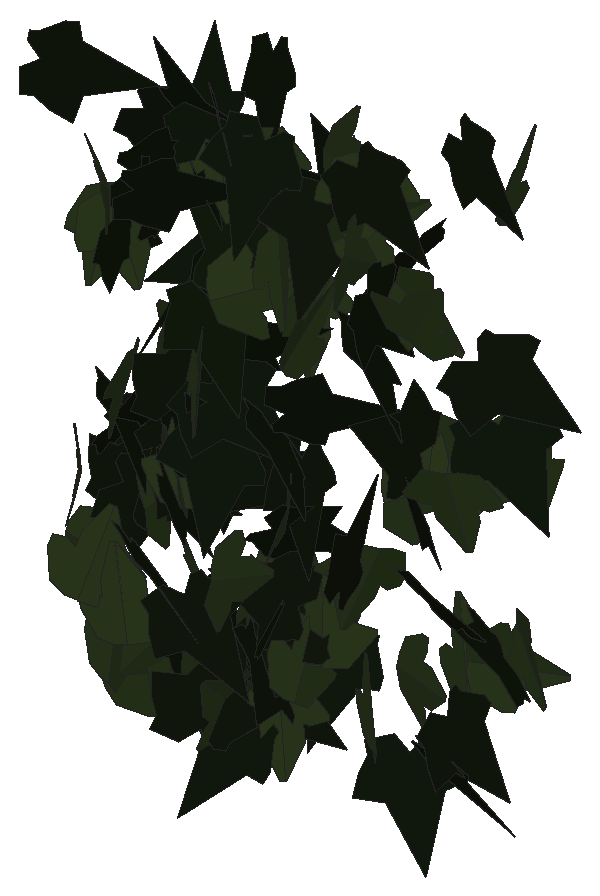
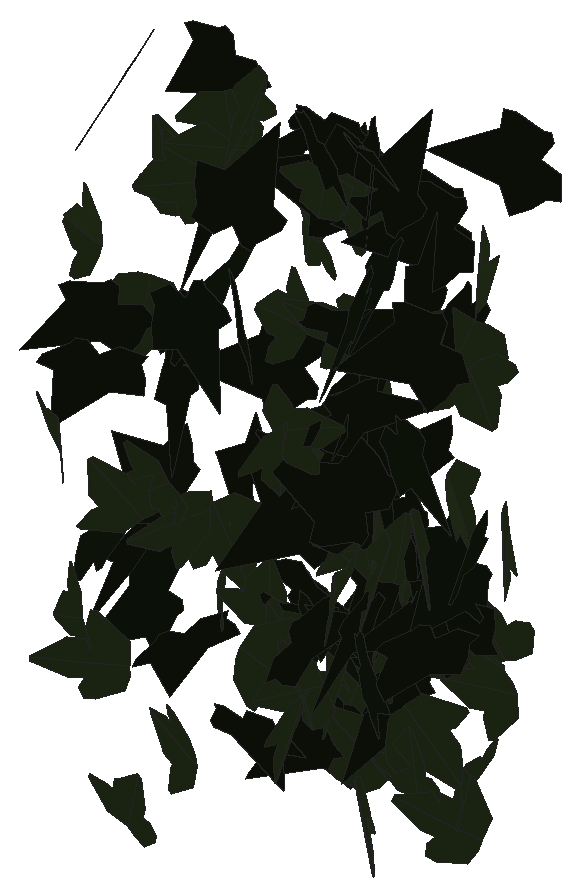
# SketchUp Ruby script. Lengths in inches.
U = 1.inch
M = Sketchup.active_model
def pt(a) = Geom::Point3d.new(a.map { |v| v * U })
def face(e, loops, mat)
  f = e.add_face(loops[0].map { |a| pt(a) })
  loops[1..].each { |l| e.add_face(l.map { |a| pt(a) }).erase! }
  f.material = f.back_material = mat if mat
  f
end
# faces: each face lists its corners as indices into pts; further lists are holes
def faces(e, pts, list, mat = nil) = list.each { |f| face(e, (f[0].is_a?(Array) ? f : [f]).map { |l| l.map { |i| pts[i] } }, mat) }
# xy, xz, yz: faces in a plane at the given z, y or x. An outline is a flat list of corners, or four numbers for a rectangle; further outlines are holes
def ring(l) = l.size == 4 ? [[l[0], l[1]], [l[2], l[1]], [l[2], l[3]], [l[0], l[3]]] : l.each_slice(2).to_a
def flat(e, list, mat, &to3) = list.each { |f| face(e, (f[0].is_a?(Array) ? f : [f]).map { |l| ring(l).map { |u, v| to3.(u, v) } }, mat) }
def xy(e, z, list, mat = nil) = flat(e, list, mat) { |x, y| [x, y, z] }
def xz(e, y, list, mat = nil) = flat(e, list, mat) { |x, z| [x, y, z] }
def yz(e, x, list, mat = nil) = flat(e, list, mat) { |y, z| [x, y, z] }
def lines(e, pts, list) = list.each { |a, b| e.add_line(pt(pts[a]), pt(pts[b])) }
# prism: a flat outline (further loops are holes) pulled along v
def prism(e, loops, v, mat = nil)
  f = face(e, loops, mat); d = Geom::Vector3d.new(v.map { |x| x * U })
  f.pushpull(f.normal.samedirection?(d) ? d.length : -d.length)
end
def box(e, o, s, mat = nil) = prism(e, [[o, [o[0] + s[0], o[1], o[2]], [o[0] + s[0], o[1] + s[1], o[2]], [o[0], o[1] + s[1], o[2]]]], [0, 0, s[2]], mat)
def at(x, y, z, deg = 0) = Geom::Transformation.translation(pt([x, y, z])) * Geom::Transformation.rotation(ORIGIN, Z_AXIS, deg.degrees)
def axes(o, x, y, z) = Geom::Transformation.new([*x, 0, *y, 0, *z, 0, *pt(o).to_a, 1])
def part(name) = M.definitions.add(name)
# library, detail: a bought-in or finely detailed component or shape, given as its bounding box
def library(name, o, s) = part(name).tap { |d| box(d.entities, o, s) }
def detail(e, o, s) = box(e.add_group.entities, o, s)
def put(e, d, t, mat = nil) = e.add_instance(d, t).tap { |i| i.material = mat if mat }
def group(e, t, mat = nil) = e.add_group.tap { |g| g.transformation = t; g.material = mat if mat }.entities
root = M.entities
M.materials.add("efeu1").color = [18, 25, 13]
M.materials.add("efeu2").color = [43, 57, 29]
c1 = part("ivyleaf_9")
p = [[1.54,2.16,1.25],[1.36,2.04,1.19],[-0.21,0.99,0.68],[-0.71,1.11,0.82],[-0.85,0.86,0.67],[-0.8,0.17,0.21],
  [-0.9,-0.01,0.1],[-0.67,-0.16,-0.02],[-0.08,-0.08,-0.05],[-0.03,-0.6,-0.4],[0.65,-0.88,-0.66],[0.83,-0.6,-0.49],
  [1.29,-0.42,-0.43],[1.8125,-0.07,-0.26],[1.21,0.44,0.15]]
faces(c1.entities,p,[[0,1,2,3,4,5,6,7,8,9,10,11,12,13,14]],"efeu1")
c2 = part("ivyleaf_10")
p = [[0,0.5,-0.03],[-0.0625,2.02,-0.43],[-0.19,2.01,-0.46],[-0.54,1.05,-0.29],[-0.52,0.625,-0.18],[-0.83,0.76,-0.28],
  [-1.16,0.64,-0.33],[-1.15,0.33,-0.24],[-0.77,-0.39,0.02],[-0.3,-0.51,0.16],[0.04,-0.48,0.23],[-0.02,2.01,-0.4375],
  [-0.06,2.01,-0.43],[0.04,-0.49,0.23],[0.67,-0.49,0.14],[1.38,0.36,-0.2],[1.375,0.51,-0.24],[0.81,0.65,-0.19],
  [0.62,0.59,-0.15],[0.6,1.09,-0.28],[0.5,1.23,-0.31]]
faces(c2.entities,p,[[0,1,2,3,4,5,6,7,8,9,10],[11,12,0,13,14,15,16,17,18,19,20]],"efeu2")
put(root,c1,axes([37.89,224.72,217.01],[0.06828,-0.29267,-0.3996],[0.02885,0.40505,-0.29173],[0.49447,0.01679,0.0722]))
put(root,c2,axes([38.07,223.66,220.32],[0.25896,0.39819,-0.15615],[-0.07769,-0.13571,-0.47492],[-0.4206,0.27023,-0.00841]))
put(root,c2,axes([38.36,223.23,214.16],[0.00126,0.31534,-0.38802],[-0.07703,0.38351,0.31143],[0.49403,0.05899,0.04955]))
put(root,c2,axes([37.9,223.36,215.67],[-0.1061,-0.00591,-0.48858],[0.46752,-0.14654,-0.09976],[-0.14201,-0.47801,0.03662]))
put(root,c2,axes([38.43,224.34,218.27],[0.23981,-0.31066,-0.30981],[-0.16582,0.26271,-0.39178],[0.4062,0.29065,0.02298]))
put(root,c1,axes([38.34,223.5,217.45],[0.13194,0.388,0.28644],[0.09321,0.27085,-0.40982],[-0.47318,0.16154,-0.00086]))
put(root,c1,axes([37.98,224.53,221.21],[0.05891,0.07528,-0.49078],[0.31473,0.37659,0.09554],[0.38402,-0.32018,-0.00302]))
put(root,c1,axes([38.24,225.7,216.92],[-0.25111,0.04925,-0.42955],[0.39721,-0.16992,-0.25169],[-0.17078,-0.46765,0.04621]))
put(root,c2,axes([38.59,222.34,217.34],[0.11945,-0.23218,-0.42641],[-0.16922,0.39168,-0.26068],[0.45508,0.20659,0.01499]))
put(root,c1,axes([38.09,222.35,222.93],[0.22534,0.05977,-0.44232],[0.26473,0.38104,0.18635],[0.35936,-0.31818,0.14008]))
put(root,c1,axes([38.19,223.74,217.46],[0.16614,-0.37636,0.28417],[0.11736,-0.25881,-0.41139],[0.45675,0.2034,0.00235]))
put(root,c2,axes([38.18,223.69,213.68],[-0.11724,-0.15903,0.45931],[0.41144,0.21909,0.18088],[-0.25879,0.42037,0.07949]))
put(root,c2,axes([38.56,223.4,218.38],[0.19224,-0.45308,0.08813],[0.04208,-0.07787,-0.4921],[0.45965,0.19662,0.00819]))
put(root,c1,axes([38.45,223.53,216.39],[-0.3181,0.09077,0.37494],[0.31904,-0.21129,0.32182],[0.21686,0.44398,0.07651]))
put(root,c2,axes([38.53,222.94,221.02],[-0.266,0.14555,0.39757],[0.31073,-0.25179,0.30008],[0.28756,0.40672,0.0435]))
put(root,c2,axes([38.57,222.53,215.71],[0.40715,0.22638,-0.1816],[0.15911,0.08754,0.46586],[0.24271,-0.43714,-0.00075]))
put(root,c1,axes([38.8,222.83,220.69],[0.06508,-0.02692,-0.49502],[-0.34481,0.35626,-0.0647],[0.35619,0.34979,0.02781]))
put(root,c1,axes([38.87,224.16,219.36],[-0.33398,0.30789,-0.20895],[0.15546,-0.13964,-0.45424],[-0.33807,-0.36838,-0.00246]))
put(root,c2,axes([38.52,223.15,220.61],[0.41422,0.19482,0.20116],[0.17576,0.09875,-0.45755],[-0.21801,0.44977,0.01332]))
put(root,c1,axes([38.5,223.47,216.62],[0.12107,0.03791,-0.48364],[0.13119,0.47734,0.07025],[0.46705,-0.1439,0.10563]))
put(root,c2,axes([38.95,224.82,214.375],[0.18786,-0.30213,-0.35132],[-0.19064,0.29513,-0.35574],[0.42233,0.26761,-0.00431]))
put(root,c2,axes([38.81,223.55,216.45],[0.12865,-0.02468,-0.48253],[0.0261,0.49897,-0.01856],[0.48246,-0.02041,0.12968]))
put(root,c2,axes([39.14,223.51,214.83],[-0.30526,-0.23645,0.31766],[-0.25376,-0.19111,-0.38611],[0.30401,-0.39695,-0.00333]))
put(root,c2,axes([39.12,222.64,215.25],[0.44305,0.21822,0.078],[-0.07088,-0.03261,0.49387],[0.22064,-0.44868,0.00204]))
put(root,c2,axes([39.08,223.61,213.99],[0.49527,-0.04984,0.04714],[-0.04691,0.00468,0.49777],[-0.05006,-0.49749,-0.00004]))
put(root,c2,axes([39.3,224.87,217.23],[-0.06855,0.33915,-0.36094],[-0.1058,0.34595,0.34515],[0.48385,0.1237,0.02434]))
put(root,c1,axes([39.11,223.39,220.84],[0.03874,0.18578,0.46258],[-0.14418,-0.43997,0.18878],[0.47719,-0.14802,0.01948]))
put(root,c1,axes([39.12,224.59,221.51],[0.34556,-0.18671,-0.30941],[-0.27171,0.14801,-0.39277],[0.23826,0.43958,0.00083]))
put(root,c2,axes([39.24,223.51,216.83],[-0.40564,0.28083,0.08119],[0.06484,-0.04899,0.49335],[0.28505,0.41078,0.00332]))
put(root,c1,axes([39.25,224.4,216.82],[0.19395,-0.12326,-0.44406],[-0.29917,0.33279,-0.22304],[0.35054,0.35222,0.05534]))
put(root,c1,axes([39.44,224.75,219.78],[-0.00126,-0.22965,-0.44414],[-0.02405,-0.4436,0.22944],[-0.49942,0.02194,-0.00993]))
put(root,c1,axes([39.28,223.24,217.05],[0.35864,-0.15511,-0.31196],[-0.27416,0.15061,-0.39007],[0.21498,0.45084,0.02298]))
put(root,c2,axes([39.49,223.77,217.21],[-0.14057,0.22616,0.42319],[-0.24515,0.34523,-0.26593],[-0.41248,-0.28225,0.01383]))
put(root,c1,axes([38.96,223.63,217.67],[0.15554,-0.09957,-0.46464],[0.47489,0.04995,0.14826],[0.01689,-0.48743,0.11011]))
put(root,c1,axes([39.49,223.4375,215.13],[-0.00738,0.01927,-0.49957],[-0.28837,0.40797,0.02],[0.4084,0.28842,0.00509]))
put(root,c1,axes([39.24,222.68,221.64],[0.07634,0.2977,-0.39439],[0.01251,0.39778,0.30268],[0.49398,-0.05608,0.05328]))
put(root,c2,axes([39.47,223.47,216.93],[0.41651,0.2713,0.05402],[-0.05339,-0.01696,0.49685],[0.27142,-0.41965,0.01483]))
put(root,c1,axes([39.5,223.77,220.15],[0.15808,-0.0587,-0.47071],[-0.34269,0.32893,-0.15611],[0.32799,0.37197,0.06377]))
put(root,c1,axes([39.17,222.78,216.24],[0.35133,-0.32097,0.15346],[0.11135,-0.10563,-0.47586],[0.33789,0.36854,-0.00274]))
put(root,c2,axes([39.78,223.34,215.58],[-0.16886,0.26984,-0.38558],[-0.28503,0.26734,0.31191],[0.3745,0.32514,0.06354]))
put(root,c1,axes([39.5,223.19,218.27],[-0.21601,-0.16653,0.41906],[0.35664,0.22125,0.27176],[-0.27595,0.41631,0.0232]))
put(root,c2,axes([39.73,223.52,217.81],[0.08641,-0.21543,-0.44286],[-0.15294,0.41565,-0.23204],[0.46813,0.17556,0.00594]))
put(root,c1,axes([39.22,224.52,218.375],[0.15788,-0.11672,0.45984],[0.47304,0.00175,-0.16197],[0.0362,0.48618,0.11098]))
put(root,c1,axes([39.61,223.43,221.54],[0.36266,-0.09615,-0.3305],[-0.30475,0.13351,-0.37324],[0.16002,0.47216,0.03823]))
put(root,c1,axes([39.72,223.42,222.14],[0.32429,-0.25113,0.28595],[-0.22912,0.17114,0.41014],[-0.30387,-0.39704,-0.00408]))
put(root,c1,axes([39.65,225.32,216.64],[0.06197,-0.19463,-0.45637],[0.18227,-0.41883,0.20337],[-0.46145,-0.19158,0.01905]))
put(root,c2,axes([39.77,225.17,215.51],[-0.1374,0.47457,0.07683],[-0.02529,0.07266,-0.49404],[-0.48009,-0.13965,0.00404]))
put(root,c2,axes([40.13,224.89,219.35],[0.21577,0.04384,0.44891],[-0.43819,-0.09758,0.22015],[0.10691,-0.48842,-0.00369]))
put(root,c1,axes([39.52,222.41,221.57],[0.11285,0.25711,-0.41372],[0.17466,0.37507,0.28074],[0.45471,-0.20788,-0.00516]))
put(root,c1,axes([39.91,223.71,217.39],[0.22814,0.14471,0.42073],[-0.35434,-0.22684,0.27016],[0.26906,-0.42143,-0.00095]))
put(root,c1,axes([40.06,223.05,222.29],[-0.45252,0.20011,-0.07197],[-0.07166,0.01582,0.49459],[0.20021,0.45794,0.01437]))
put(root,c1,axes([40.26,223.8,220.29],[-0.40551,-0.24372,-0.16174],[-0.13937,-0.08209,0.47311],[-0.25717,0.42879,-0.00136]))
put(root,c2,axes([39.74,223.57,214.07],[-0.28617,-0.19014,0.36325],[0.33377,0.14924,0.34106],[-0.23812,0.43769,0.04151]))
put(root,c1,axes([39.93,223.28,219.76],[0.05276,-0.46715,-0.17027],[-0.00403,0.17082,-0.4699],[0.49719,0.05096,0.01426]))
put(root,c2,axes([39.92,223.0625,219.1],[0.24328,-0.22779,0.37273],[0.29412,-0.23002,-0.33254],[0.32297,0.38105,0.02207]))
put(root,c1,axes([40.0625,223.32,217.83],[-0.11167,-0.48727,-0.00989],[0.00254,0.00956,-0.4999],[0.48736,-0.1117,0.00034]))
put(root,c1,axes([39.96,223.36,218.54],[0.07325,-0.25074,-0.42634],[0.09462,0.43013,-0.23671],[0.48547,-0.046,0.11046]))
put(root,c2,axes([39.99,224.81,215.74],[0.26972,-0.21404,0.36254],[0.30068,-0.20345,-0.3438],[0.2947,0.40348,0.01897]))
put(root,c1,axes([40.44,222.86,222.58],[0.16918,0.02978,-0.46956],[-0.46422,0.09188,-0.16143],[0.07668,0.49058,0.05874]))
put(root,c2,axes([40.1,223.28,222.08],[0.46778,0.11724,0.13204],[0.12646,0.03848,-0.48221],[-0.12323,0.48454,0.00635]))
put(root,c2,axes([40.23,224.875,219.23],[0.06428,0.48943,-0.07953],[-0.01742,-0.07792,-0.49358],[-0.49554,0.06623,0.00703]))
put(root,c2,axes([39.93,224.64,215.58],[0.22817,0.02231,0.44435],[0.42706,0.12904,-0.22577],[-0.12475,0.48255,0.03983]))
put(root,c2,axes([40.39,223.42,215.23],[-0.23851,0.42044,0.12785],[-0.06564,0.10975,-0.48337],[-0.43452,-0.24736,0.00284]))
put(root,c1,axes([40.16,222.54,215.98],[-0.10432,-0.17674,-0.45594],[0.338,0.31084,-0.19783],[0.35337,-0.34949,0.05462]))
put(root,c1,axes([40.375,223.95,223.07],[-0.28216,-0.03138,-0.41158],[0.41249,-0.00271,-0.28257],[0.0155,-0.49901,0.02742]))
put(root,c1,axes([40.49,222.43,214.4],[-0.31875,-0.07522,0.37781],[0.37636,0.04381,0.32625],[-0.08219,0.49236,0.02869]))
put(root,c1,axes([40.74,223.03,214.2],[-0.48845,-0.09028,-0.05712],[0.05664,0.00782,-0.49672],[0.09058,-0.49172,0.00259]))
put(root,c1,axes([40.34,223.57,214.42],[-0.00983,-0.04775,-0.49762],[0.21621,0.44835,-0.04729],[0.45073,-0.21611,0.01184]))
put(root,c2,axes([40.29,223.24,220.03],[0.16619,0.01862,-0.47121],[0.45398,0.12889,0.16521],[0.12762,-0.48274,0.02594]))
put(root,c2,axes([40.67,222.87,214.51],[-0.12754,-0.31785,-0.36429],[-0.06786,-0.36125,0.33896],[-0.47867,0.1359,0.04901]))
put(root,c1,axes([40.96,224.74,220.5],[-0.01077,0.08581,0.49246],[-0.07654,0.48649,-0.08644],[-0.49399,-0.07725,0.00265]))
put(root,c1,axes([41.24,223.31,215.95],[-0.26531,0.16174,0.39173],[-0.33882,0.19667,-0.31068],[-0.25459,-0.4303,0.00525]))
put(root,c2,axes([40.65,223.41,222.11],[0.46483,0.09359,0.15865],[0.15567,0.03061,-0.47416],[-0.09847,0.49021,-0.00068]))
put(root,c1,axes([41.02,223.24,215.83],[-0.35931,0.25015,-0.2415],[0.19262,-0.14592,-0.43773],[-0.28947,-0.40759,0.00849]))
put(root,c2,axes([40.89,222.3125,216.64],[0.029,-0.19135,-0.46102],[0.12408,0.45007,-0.179],[0.48349,-0.10403,0.07359]))
put(root,c1,axes([40.97,224.69,214.74],[-0.43283,-0.16937,-0.18431],[0.17294,0.06382,-0.46478],[0.18097,-0.46609,0.00334]))
put(root,c1,axes([40.54,223.08,221.89],[0.24717,-0.06967,0.42901],[0.4268,-0.05436,-0.25473],[0.08214,0.49213,0.0326]))
put(root,c1,axes([41.39,223.17,215.32],[-0.47964,-0.06391,-0.12596],[-0.12354,-0.02629,0.48378],[-0.06846,0.4952,0.00943]))
put(root,c1,axes([41.13,222.82,222.59],[-0.40535,-0.19644,-0.21703],[0.19412,0.09708,-0.45044],[0.2191,-0.44943,-0.00244]))
put(root,c1,axes([40.96,223.17,215.0625],[0.00558,-0.31516,0.38813],[0.07567,-0.38315,-0.3122],[0.49421,0.06222,0.04342]))
put(root,c2,axes([41.22,224.18,215.36],[-0.00987,-0.34879,0.35811],[0.00482,-0.35823,-0.34878],[0.49988,-0.00343,0.01043]))
put(root,c2,axes([41.08,223.16,214.63],[0.46179,0.15625,0.11107],[0.10649,0.0318,-0.48749],[-0.1594,0.4739,-0.00391]))
put(root,c1,axes([40.96,223.28,218.24],[0.15372,-0.39208,0.26952],[0.15448,-0.22676,-0.41799],[0.45001,0.21178,0.05142]))
put(root,c1,axes([41.16,223.08,217.09],[0.37557,0.24576,0.22034],[0.18437,0.12065,-0.44883],[-0.27378,0.41838,0]))
put(root,c2,axes([41.17,223.01,221.07],[0.34868,-0.14097,0.32947],[0.30334,-0.12864,-0.37608],[0.1908,0.46214,-0.00418]))
put(root,c1,axes([41.24,223.44,217.875],[-0.24087,-0.13466,-0.41695],[0.42346,0.05067,-0.26099],[0.11254,-0.47885,0.08963]))
put(root,c2,axes([41.45,223.08,219.66],[0.1167,-0.31584,0.36963],[-0.11179,0.35252,0.3365],[-0.47317,-0.16118,0.01166]))
put(root,c2,axes([41.47,223.07,215.0625],[0.08629,0.3937,-0.29589],[0.07725,0.28586,0.40288],[0.4864,-0.11525,-0.01149]))
put(root,c2,axes([41.625,226.26,213.8],[0.4574,-0.02992,0.19974],[-0.19729,0.03962,0.45772],[-0.04322,-0.49753,0.02444]))
put(root,c2,axes([41.6875,222.55,217.77],[0.11945,-0.35906,-0.32681],[-0.12305,0.30318,-0.37807],[0.46967,0.17075,-0.01593]))
put(root,c1,axes([41.71,223.98,221.49],[0.3484,-0.12266,0.33701],[-0.31024,0.13264,0.369],[-0.17992,-0.46622,0.01632]))
put(root,c2,axes([41.63,223.39,215.48],[0.48325,0.12023,0.04493],[-0.04501,-0.00517,0.49794],[0.1202,-0.4853,0.00583]))
put(root,c1,axes([41.91,224.7,220.52],[-0.14755,0.45522,-0.14494],[0.04689,-0.13716,-0.47853],[-0.47543,-0.15481,-0.00222]))
put(root,c2,axes([41.54,225.21,214.28],[0.03594,-0.02461,-0.4981],[0.38676,-0.31389,0.04342],[-0.31484,-0.38841,-0.00353]))
put(root,c1,axes([41.52,222.89,218.93],[0.28369,0.04941,0.40875],[0.39797,0.09435,-0.28761],[-0.10555,0.48852,0.01421]))
put(root,c1,axes([41.97,222.99,221.91],[-0.14545,-0.47755,0.02807],[-0.0052,-0.02776,-0.4992],[0.47835,-0.1455,0.00311]))
put(root,c2,axes([42.17,222.97,222.74],[-0.11563,0.29128,0.38959],[-0.16963,0.35117,-0.3129],[-0.45591,-0.20454,0.01761]))
put(root,c2,axes([42.22,223.62,216.75],[-0.22524,-0.41127,0.17356],[-0.07403,-0.1573,-0.4688],[0.44021,-0.23689,0.00997]))
put(root,c2,axes([41.99,224.43,217.25],[0.08121,-0.06009,-0.48969],[0.25073,0.43244,-0.01149],[0.4249,-0.24369,0.10037]))
put(root,c1,axes([42.4,222.77,216.88],[0.00833,-0.1021,0.48939],[0.15221,0.46674,0.09479],[-0.4762,0.1474,0.03885]))
put(root,c2,axes([42.18,224.88,217.84],[0.28455,0.05625,0.40727],[0.40383,0.05471,-0.2897],[-0.07715,0.4938,-0.0143]))
put(root,c2,axes([42.5,223.11,222.54],[0.38567,0.31458,-0.04794],[-0.03704,-0.03043,-0.4977],[-0.31605,0.38745,-0.00017]))
put(root,c1,axes([42.35,223.32,220.03],[0.23071,-0.41014,0.16897],[0.08323,-0.14705,-0.47058],[0.43571,0.24527,0.00042]))
put(root,c2,axes([42.51,222.89,221.77],[-0.03051,-0.16127,0.47229],[0.14121,0.45105,0.16314],[-0.47867,0.14334,0.01802]))
put(root,c2,axes([42.57,224.96,217.41],[0.32564,0.24396,-0.29058],[0.2323,0.17457,0.40689],[0.29999,-0.40001,0.00035]))
put(root,c1,axes([42.84,222.78,221.09],[0.17481,-0.17311,-0.43529],[-0.31275,0.30277,-0.24601],[0.34875,0.35828,-0.00242]))
put(root,c2,axes([43.06,222.51,215.14],[-0.1373,0.26874,-0.39866],[-0.17309,0.35917,0.30173],[0.44854,0.22086,-0.0056]))
put(root,c2,axes([42.93,222.24,221.94],[0.06126,-0.28343,-0.40733],[-0.00533,0.41002,-0.2861],[0.4962,0.0394,0.04722]))
put(root,c2,axes([42.97,225.33,221.34],[0.19216,-0.31756,0.33501],[-0.16179,0.29352,0.37104],[-0.43232,-0.251,0.01005]))
put(root,c1,axes([42.82,222.625,222.89],[-0.06366,-0.10456,-0.48478],[0.40064,0.27723,-0.1124],[0.2923,-0.40276,0.04849]))
put(root,c1,axes([43.26,223.19,218.86],[-0.05262,0.03724,0.49583],[-0.2607,-0.42663,0.00437],[0.4234,-0.25807,0.06432]))
put(root,c1,axes([43.41,222.93,218.35],[0.27148,0.01476,-0.41962],[-0.41875,0.04618,-0.26929],[0.03081,0.49764,0.03744]))
put(root,c1,axes([43.18,223.15,214.55],[-0.04944,-0.46795,-0.16905],[0.01663,0.16824,-0.47055],[0.49727,-0.05215,-0.00107]))
put(root,c2,axes([42.99,224.91,214.99],[0.00814,-0.02543,0.49929],[0.38148,0.32306,0.01023],[-0.32312,0.38077,0.02466]))
put(root,c2,axes([43.23,223.02,221.09],[0.18694,-0.0298,0.46278],[0.45981,0.07671,-0.1808],[-0.06023,0.49318,0.05608]))
put(root,c2,axes([43.49,222.85,220.77],[-0.43398,-0.10869,0.22325],[0.22421,0.02166,0.44639],[-0.10671,0.48756,0.02994]))
put(root,c1,axes([43.55,223.77,223.02],[0.31659,-0.29889,-0.24583],[-0.15676,0.19134,-0.43453],[0.35383,0.35221,0.02744]))
put(root,c1,axes([43.33,223.37,216.68],[0.11401,-0.27199,0.40376],[0.32529,-0.26596,-0.27101],[0.3622,0.32448,0.11631]))
put(root,c2,axes([43.89,224.87,217.81],[0.34606,-0.20713,0.29553],[-0.25299,0.15276,0.40331],[-0.25736,-0.42868,0.00093]))
put(root,c1,axes([43.48,224.2,219.72],[0.08072,-0.14619,-0.47129],[0.18858,0.45044,-0.10742],[0.45598,-0.16041,0.12785]))
put(root,c2,axes([43.46,224.9375,215.5],[0.17212,-0.10054,0.45855],[0.43917,-0.13804,-0.19512],[0.16583,0.46993,0.04079]))
put(root,c1,axes([43.73,224.24,218.89],[-0.11702,-0.30536,-0.37824],[0.15478,0.34539,-0.32672],[0.46081,-0.19355,0.01369]))
put(root,c1,axes([43.7,222.91,214.89],[0.4836,-0.11255,0.05882],[0.05648,-0.01678,-0.49652],[0.11374,0.48688,-0.00351]))
put(root,c1,axes([43.92,224.03,215.83],[0.33115,-0.36378,-0.08947],[0.06072,-0.06571,0.49193],[-0.36967,-0.33667,0.00066]))
put(root,c2,axes([44.22,222.66,218.94],[-0.4737,-0.15187,-0.05044],[0.04829,0.0146,-0.49745],[0.15257,-0.47615,0.00084]))
put(root,c1,axes([44.125,222.76,215.58],[0.19044,-0.2784,-0.36908],[-0.17175,0.328,-0.33603],[0.42922,0.25477,0.0293]))
